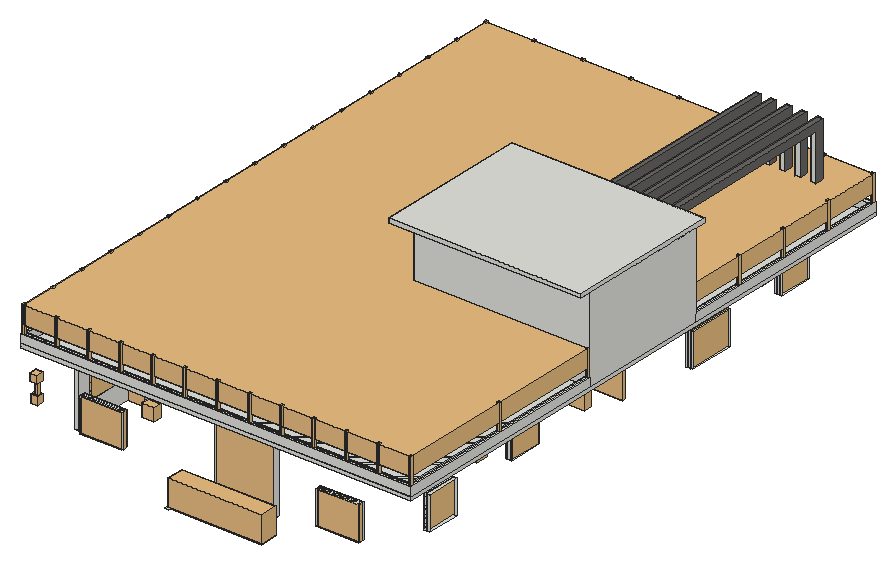
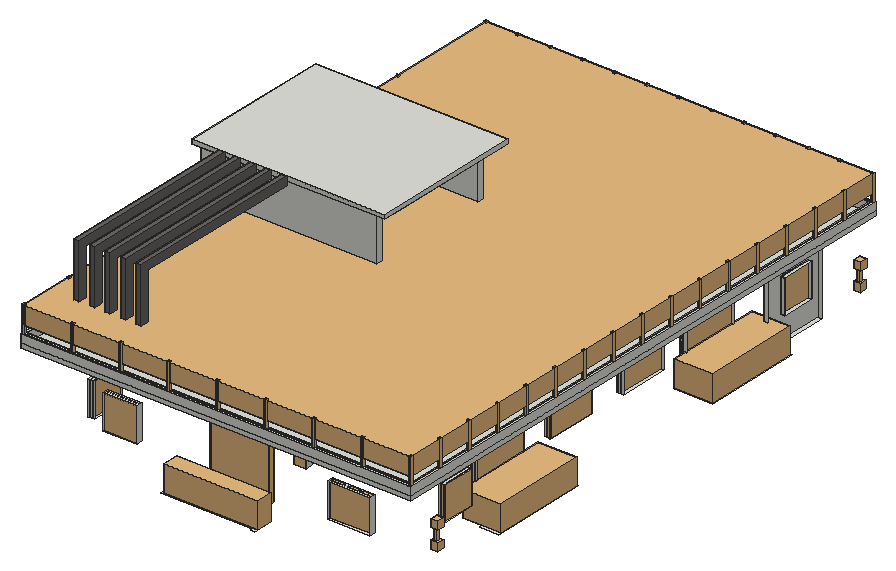
# SketchUp Ruby script. Lengths in inches.
U = 1.inch
M = Sketchup.active_model
def pt(a) = Geom::Point3d.new(a.map { |v| v * U })
def face(e, loops, mat)
  f = e.add_face(loops[0].map { |a| pt(a) })
  loops[1..].each { |l| e.add_face(l.map { |a| pt(a) }).erase! }
  f.material = f.back_material = mat if mat
  f
end
# faces: each face lists its corners as indices into pts; further lists are holes
def faces(e, pts, list, mat = nil) = list.each { |f| face(e, (f[0].is_a?(Array) ? f : [f]).map { |l| l.map { |i| pts[i] } }, mat) }
# xy, xz, yz: faces in a plane at the given z, y or x. An outline is a flat list of corners, or four numbers for a rectangle; further outlines are holes
def ring(l) = l.size == 4 ? [[l[0], l[1]], [l[2], l[1]], [l[2], l[3]], [l[0], l[3]]] : l.each_slice(2).to_a
def flat(e, list, mat, &to3) = list.each { |f| face(e, (f[0].is_a?(Array) ? f : [f]).map { |l| ring(l).map { |u, v| to3.(u, v) } }, mat) }
def xy(e, z, list, mat = nil) = flat(e, list, mat) { |x, y| [x, y, z] }
def xz(e, y, list, mat = nil) = flat(e, list, mat) { |x, z| [x, y, z] }
def yz(e, x, list, mat = nil) = flat(e, list, mat) { |y, z| [x, y, z] }
def lines(e, pts, list) = list.each { |a, b| e.add_line(pt(pts[a]), pt(pts[b])) }
# prism: a flat outline (further loops are holes) pulled along v
def prism(e, loops, v, mat = nil)
  f = face(e, loops, mat); d = Geom::Vector3d.new(v.map { |x| x * U })
  f.pushpull(f.normal.samedirection?(d) ? d.length : -d.length)
end
def box(e, o, s, mat = nil) = prism(e, [[o, [o[0] + s[0], o[1], o[2]], [o[0] + s[0], o[1] + s[1], o[2]], [o[0], o[1] + s[1], o[2]]]], [0, 0, s[2]], mat)
def at(x, y, z, deg = 0) = Geom::Transformation.translation(pt([x, y, z])) * Geom::Transformation.rotation(ORIGIN, Z_AXIS, deg.degrees)
def axes(o, x, y, z) = Geom::Transformation.new([*x, 0, *y, 0, *z, 0, *pt(o).to_a, 1])
def part(name) = M.definitions.add(name)
# library, detail: a bought-in or finely detailed component or shape, given as its bounding box
def library(name, o, s) = part(name).tap { |d| box(d.entities, o, s) }
def detail(e, o, s) = box(e.add_group.entities, o, s)
def put(e, d, t, mat = nil) = e.add_instance(d, t).tap { |i| i.material = mat if mat }
def group(e, t, mat = nil) = e.add_group.tap { |g| g.transformation = t; g.material = mat if mat }.entities
root = M.entities
M.materials.add("Stone C 250cm").color = [107, 104, 102]
c1 = library("Group\#21",[0,0,0],[134.45,23.44,36.98])
c2 = library("Window Crafter Sliding",[0,-0.55,0],[84,4.49,96])
c3 = library("Group\#18",[0,0,0],[54.77,134.11,36.98])
c4 = library("Group\#23",[0,0,0],[133.24,24.34,36.98])
c5 = library("Group\#17",[0,0,0],[54.54,138.15,36.98])
c6 = library("Group\#6",[0,0,0],[112.45,3.15,94.27])
c7 = library("Group\#11",[0,0,0],[103.79,11.15,157.27])
c8 = library("Window Crafter Sliding 6",[0,-0.55,0],[72,4.49,48])
c9 = library("Window Crafter Sliding 2",[0,-0.55,0],[48,4.49,48])
c10 = library("Window Crafter Sliding 5",[0,-0.55,0],[66,4.49,48])
c11 = library("Window Crafter Sliding 3",[0,-0.55,0],[60,4.49,48])
c12 = library("Spot Light\#1",[-5.1,-5.1,-11.05],[10.2,10.2,11.05])
c13 = library("Lamp Wall Outdoor 94-02",[-1.89,-4.65,-3.17],[3.78,4.65,6.35])
c14 = library("Group\#12",[0,0,0],[113.66,3.15,100.57])
c15 = library("Window Crafter Awning 2",[0,-9.5,0],[17.5,11.27,18])
c16 = library("Tlon Light 650 Ceiling 152 007",[-12.8,-12.8,-3.78],[25.6,25.6,3.58])
c17 = part("Square rail bar")
box(c17.entities,[0,0,-1],[51.7,1,1])
c18 = part("Group\#20")
xy(c18.entities,0,[[0,0,51.7,106.6]])
xy(c18.entities,1,[[0,0,51.7,107.6]])
xz(c18.entities,0,[[0,0,51.7,1]])
xz(c18.entities,107.6,[[0,0,51.7,1]])
yz(c18.entities,0,[[0,0,107.6,1]])
yz(c18.entities,51.7,[[0,0,107.6,1]])
put(c18.entities,c17,at(0,106.6,0))
put(c18.entities,c17,at(0,0,0))
put(c18.entities,c17,at(0,103.05,0))
put(c18.entities,c17,at(0,99.49,0))
put(c18.entities,c17,at(0,95.94,0))
put(c18.entities,c17,at(0,92.39,0))
put(c18.entities,c17,at(0,88.83,0))
put(c18.entities,c17,at(0,85.28,0))
put(c18.entities,c17,at(0,81.73,0))
put(c18.entities,c17,at(0,78.17,0))
put(c18.entities,c17,at(0,74.62,0))
put(c18.entities,c17,at(0,71.07,0))
put(c18.entities,c17,at(0,67.51,0))
put(c18.entities,c17,at(0,63.96,0))
put(c18.entities,c17,at(0,60.41,0))
put(c18.entities,c17,at(0,56.85,0))
put(c18.entities,c17,at(0,53.3,0))
put(c18.entities,c17,at(0,49.75,0))
put(c18.entities,c17,at(0,46.19,0))
put(c18.entities,c17,at(0,42.64,0))
put(c18.entities,c17,at(0,39.09,0))
put(c18.entities,c17,at(0,35.53,0))
put(c18.entities,c17,at(0,31.98,0))
put(c18.entities,c17,at(0,28.43,0))
put(c18.entities,c17,at(0,24.875,0))
put(c18.entities,c17,at(0,21.32,0))
put(c18.entities,c17,at(0,17.77,0))
put(c18.entities,c17,at(0,14.21,0))
put(c18.entities,c17,at(0,10.66,0))
put(c18.entities,c17,at(0,7.11,0))
put(c18.entities,c17,at(0,3.55,0))
put(c18.entities,c17,at(0,0,0))
c19 = part("Opening frame")
xy(c19.entities,0,[[0,0,7.4375,12]])
xy(c19.entities,114,[[0,-246.7,7.4375,0]])
xy(c19.entities,126,[[0,-246.7,7.4375,12]],"Stone C 250cm")
xz(c19.entities,-246.7,[[0,114,7.4375,126]])
xz(c19.entities,0,[[0,0,7.4375,114]])
xz(c19.entities,12,[[0,0,7.4375,126]],"Stone C 250cm")
yz(c19.entities,0,[[0,0,0,114,-246.7,114,-246.7,126,12,126,12,0]],"Stone C 250cm")
yz(c19.entities,7.4375,[[0,0,12,0,12,126,-246.7,126,-246.7,114,0,114]],"Stone C 250cm")
c20 = library("Ploe\#3",[2336.18,686.95,516],[3.15,3.15,37.57])
c21 = part("Group1621\#2")
put(c21.entities,c20,at(0,0,0))
put(c21.entities,c20,at(0,79.49,0))
put(c21.entities,c20,at(0,158.98,0))
put(c21.entities,c20,at(0,238.46,0))
put(c21.entities,c20,at(0,317.95,0))
put(c21.entities,c20,at(-68.83,317.95,0))
put(c21.entities,c20,at(-137.65,317.95,0))
put(c21.entities,c20,at(-206.47,317.95,0))
put(c21.entities,c20,at(-275.3,317.95,0))
put(c21.entities,c20,at(-344.125,317.95,0))
put(c21.entities,c20,at(-412.95,317.95,0))
put(c21.entities,c20,at(-481.77,317.95,0))
put(c21.entities,c20,at(-550.6,317.95,0))
put(c21.entities,c20,at(-550.6,266.57,0))
put(c21.entities,c20,at(-550.6,215.2,0))
put(c21.entities,c20,at(-550.6,163.83,0))
put(c21.entities,c20,at(-550.6,112.45,0))
put(c21.entities,c20,at(-550.6,61.08,0))
put(c21.entities,c20,at(-550.6,9.7,0))
put(c21.entities,c20,at(-550.6,-41.67,0))
put(c21.entities,c20,at(-550.6,-93.05,0))
put(c21.entities,c20,at(-550.6,-144.42,0))
put(c21.entities,c20,at(-550.6,-195.8,0))
put(c21.entities,c20,at(-550.6,-247.17,0))
put(c21.entities,c20,at(-550.6,-298.55,0))
put(c21.entities,c20,at(-550.6,-349.92,0))
put(c21.entities,c20,at(-550.6,-401.3,0))
put(c21.entities,c20,at(-550.6,-452.67,0))
put(c21.entities,c20,at(-550.6,-504.05,0))
put(c21.entities,c20,at(-504.72,-504.05,0))
put(c21.entities,c20,at(-458.83,-504.05,0))
put(c21.entities,c20,at(-412.95,-504.05,0))
put(c21.entities,c20,at(-367.07,-504.05,0))
put(c21.entities,c20,at(-321.18,-504.05,0))
put(c21.entities,c20,at(-275.3,-504.05,0))
put(c21.entities,c20,at(-229.42,-504.05,0))
put(c21.entities,c20,at(-183.53,-504.05,0))
put(c21.entities,c20,at(-137.65,-504.05,0))
put(c21.entities,c20,at(-91.77,-504.05,0))
put(c21.entities,c20,at(-45.88,-504.05,0))
put(c21.entities,c20,at(0,-504.05,0))
put(c21.entities,c20,at(0,-346.67,0))
put(c21.entities,c20,at(0,-189.3,0))
c22 = library("Group1622\#2",[1786.37,183.69,527.61],[552.17,823.58,25.18])
xy(root,381,[[2005.02,473.67,2011.02,473.67,2011.02,476.67,2141.52,476.67,2141.52,500.67,2138.32,500.67,2138.32,479.88,2008.23,479.88,2008.23,500.67,2005.02,500.67],[2008.23,479.88,2138.32,479.88,2138.32,500.67,2135.52,500.67,2135.52,482.67,2011.02,482.67,2011.02,500.67,2008.23,500.67],[2031.27,530.62,2115.27,539.67],[1789.02,637.17,1816.02,637.17,1816.02,640.17,1792.02,640.17,1792.02,775.17,1843.02,775.17,1843.02,778.17,1789.02,778.17],[1792.02,640.17,1816.02,640.17,1816.02,643.17,1795.02,643.17,1795.02,772.17,1843.02,772.17,1843.02,775.17,1792.02,775.17],
  [1843.02,673.67,1852.02,757.67],[1789.02,1018.17,1843.02,1018.17,1843.02,1020.95,1791.8,1020.95,1791.8,1151.9,1816.02,1151.9,1816.02,1159.17,1789.02,1159.17],[1791.8,1020.95,1843.02,1020.95,1843.02,1024.17,1795.02,1024.17,1795.02,1148.67,1816.02,1148.67,1816.02,1151.9,1791.8,1151.9],[1843.02,1046.67,1852.02,1130.67],[2031.27,1256.67,2115.27,1265.67],
  [2005.02,1295.67,2011.02,1295.67,2011.02,1313.67,2135.52,1313.67,2135.52,1295.67,2141.52,1295.67,2141.52,1319.67,2011.02,1319.67,2011.02,1322.67,2005.02,1322.67],[2007.35,1298.57,2007.22,1298.59,2007.1,1298.64,2007,1298.72,2006.92,1298.82,2006.87,1298.94,2006.85,1299.07,2006.87,1299.2,2006.92,1299.32,2007,1299.42,2007.1,1299.5,2007.22,1299.55,2007.35,1299.57,2007.48,1299.55,2007.6,1299.5,2007.7,1299.42,2007.78,1299.32,2007.83,1299.2,2007.85,1299.07,2007.83,1298.94,2007.78,1298.82,2007.7,1298.72,2007.6,1298.64,2007.48,1298.59],[2007.35,1315.07,2007.22,1315.09,2007.1,1315.14,2007,1315.22,2006.92,1315.32,2006.87,1315.44,2006.85,1315.57,2006.87,1315.7,2006.92,1315.82,2007,1315.92,2007.1,1316,2007.22,1316.05,2007.35,1316.07,2007.48,1316.05,2007.6,1316,2007.7,1315.92,2007.78,1315.82,2007.83,1315.7,2007.85,1315.57,2007.83,1315.44,2007.78,1315.32,2007.7,1315.22,2007.6,1315.14,2007.48,1315.09],[2051.11,1315.07,2050.98,1315.09,2050.86,1315.14,2050.76,1315.22,2050.68,1315.32,2050.63,1315.44,2050.61,1315.57,2050.63,1315.7,2050.68,1315.82,2050.76,1315.92,2050.86,1316,2050.98,1316.05,2051.11,1316.07,2051.24,1316.05,2051.36,1316,2051.47,1315.92,2051.55,1315.82,2051.6,1315.7,2051.61,1315.57,2051.6,1315.44,2051.55,1315.32,2051.47,1315.22,2051.36,1315.14,2051.24,1315.09],[2138.64,1315.07,2138.52,1315.09,2138.39,1315.14,2138.29,1315.22,2138.21,1315.32,2138.16,1315.44,2138.14,1315.57,2138.16,1315.7,2138.21,1315.82,2138.29,1315.92,2138.39,1316,2138.52,1316.05,2138.64,1316.07,2138.77,1316.05,2138.89,1316,2139,1315.92,2139.08,1315.82,2139.13,1315.7,2139.14,1315.57,2139.13,1315.44,2139.08,1315.32,2139,1315.22,2138.89,1315.14,2138.77,1315.09]])
xy(root,381.02,[[1815.02,551.67,1820.92,647.67]])
xy(root,414,[[1863.02,500.67,1923.02,509.67],[2199.52,500.67,2259.52,509.67],[1815.02,569.57,1820.92,617.57],[1816.02,569.57,1825.02,617.57],[2297.52,569.57,2306.52,617.57],
  [2267.52,752.67,2276.52,800.67],[1843.02,797.67,1852.02,869.67],[1843.02,926.67,1852.02,998.67],[2294.52,1040.67,2303.52,1106.67],[1816.02,1172.67,1825.02,1220.67],
  [2267.52,1232.67,2276.52,1280.67],[1863.02,1286.67,1923.02,1295.67],[2195.52,1286.67,2243.52,1295.67]])
xy(root,462,[[1863.02,500.67,1923.02,509.67],[2199.52,500.67,2259.52,509.67],[1815.02,569.57,1820.92,617.57],[1816.02,569.57,1825.02,617.57],[2297.52,569.57,2306.52,617.57],
  [1954.02,596.67,1978.02,602.67],[2005.02,605.67,2011.02,635.67],[2152.02,641.67,2184.02,647.67],[2198.52,641.67,2228.52,647.67],[2267.52,710.67,2276.52,740.67],
  [2267.52,752.67,2276.52,800.67],[1966.02,767.67,2002.02,773.67],[1843.02,797.67,1852.02,869.67],[2078.52,806.67,2117.52,815.67],[2008.02,809.67,2014.02,833.67],
  [1843.02,926.67,1852.02,998.67],[2008.02,962.67,2014.02,986.67],[2078.52,980.67,2117.52,989.67],[1966.02,1022.67,2002.02,1028.67],[2294.52,1040.67,2303.52,1106.67],
  [2149.02,1121.67,2181.02,1127.67],[2195.52,1121.67,2225.52,1127.67],[2005.02,1160.17,2011.02,1190.17],[1816.02,1172.67,1825.02,1220.67],[2267.52,1190.67,2276.52,1220.67],
  [1954.02,1193.67,1978.02,1199.67],[2267.52,1232.67,2276.52,1280.67],[1863.02,1286.67,1923.02,1295.67],[2195.52,1286.67,2243.52,1295.67]])
xy(root,468,[[1953.02,500.67,1970.52,509.67],[2297.52,649.73,2306.52,667.23],[2029.77,869.67,2047.27,878.67],[2029.77,917.67,2047.27,926.67],[2294.52,1162.17,2303.52,1179.67],
  [1953.02,1286.67,1970.52,1295.67]])
xy(root,477,[[2031.27,530.62,2115.27,539.67],[1843.02,673.67,1852.02,757.67],[1843.02,1046.67,1852.02,1130.67],[2031.27,1256.67,2115.27,1265.67]])
xy(root,486,[[1953.02,500.67,1970.52,509.67],[2297.52,649.73,2306.52,667.23],[2029.77,869.67,2047.27,878.67],[2029.77,917.67,2047.27,926.67],[2294.52,1162.17,2303.52,1179.67],
  [1953.02,1286.67,1970.52,1295.67]])
xy(root,498,[[[1789.02,500.67,2011.02,500.67,2011.02,647.67,1852.02,647.67,1852.02,767.67,2072.52,767.67,2072.52,806.67,2132.52,806.67,2132.52,715.17,2066.52,715.17,2066.52,686.67,2072.52,686.67,2072.52,709.17,2132.52,709.17,2132.52,686.67,2138.52,686.67,2138.52,743.67,2158.52,743.67,2158.52,749.67,2138.52,749.67,2138.52,806.67,2324.52,806.67,2324.52,815.67,2276.52,815.67,2276.52,980.67,2330.52,980.67,2330.52,1031.67,2303.52,1031.67,2303.52,1151.7,2324.52,1151.7,2324.52,1157.7,2303.52,1157.7,2303.52,1181.67,2330.52,1181.67,2330.52,1295.67,2132.52,1295.67,2132.52,1223.67,2138.52,1223.67,2138.52,1286.67,2324.52,1286.67,2324.52,1187.67,2132.52,1187.67,2132.52,1181.67,2183.52,1181.67,2183.52,1127.67,2132.52,1127.67,2132.52,989.67,2072.52,989.67,2072.52,1028.67,1852.02,1028.67,1852.02,1148.67,2011.02,1148.67,2011.02,1256.67,2132.52,1256.67,2132.52,1265.67,2011.02,1265.67,2011.02,1295.67,1798.02,1295.67,1798.02,1286.67,1945.02,1286.67,1945.02,1193.67,2005.02,1193.67,2005.02,1157.67,1997.02,1157.67,1997.02,1154.67,1825.02,1154.67,1825.02,1253.67,1816.02,1253.67,1816.02,1148.67,1843.02,1148.67,1843.02,647.67,1816.02,647.67,1816.02,551.67,1789.02,551.67],[1852.02,773.67,1852.02,893.67,2014.02,893.67,2014.02,891.17,2017.02,891.17,2017.02,905.17,2014.02,905.17,2014.02,902.67,1852.02,902.67,1852.02,1022.67,2008.02,1022.67,2008.02,902.67,2014.02,902.67,2014.02,1022.67,2066.52,1022.67,2066.52,773.67,2014.02,773.67,2014.02,893.67,2008.02,893.67,2008.02,773.67],[2075.52,815.67,2267.52,980.67],[1798.02,509.67,1798.02,542.67,1825.02,542.67,1825.02,641.67,1997.02,641.67,1997.02,638.67,2005.02,638.67,2005.02,509.67],[2138.52,989.67,2138.52,1118.67,2146.52,1118.67,2146.52,1121.67,2294.52,1121.67,2294.52,1022.67,2321.52,1022.67,2321.52,989.67],[2189.52,1127.67,2294.52,1181.67],[1951.02,1199.67,2005.02,1286.67]],[[2135.52,500.67,2333.52,500.67,2333.52,551.67,2306.52,551.67,2306.52,701.67,2333.52,701.67,2333.52,806.67,2327.52,806.67,2327.52,707.67,2186.52,707.67,2186.52,647.67,2135.52,647.67,2135.52,539.67,2011.02,539.67,2011.02,530.62,2135.52,530.62],[2141.52,509.67,2141.52,641.67,2297.52,641.67,2297.52,542.67,2324.52,542.67,2324.52,509.67],[2192.52,647.67,2297.52,701.67]],[1945.02,509.67,1951.02,509.67,1951.02,596.67,2005.02,596.67,2005.02,602.67,1945.02,602.67],[1815.02,551.67,1820.92,647.67],[2267.52,707.67,2276.52,806.67],
  [2324.52,806.67,2333.52,815.67],[2014.02,869.67,2066.52,878.67],[2014.02,917.67,2066.52,926.67],[2066.52,1081.17,2132.52,1081.17,2132.52,1087.17,2072.52,1087.17,2072.52,1109.67,2066.52,1109.67],[2132.52,1157.67,2138.52,1181.67],
  [2267.52,1187.67,2276.52,1286.67],[1789.02,1244.67,1816.02,1244.67,1816.02,1253.67,1798.02,1253.67,1798.02,1295.67,1789.02,1295.67]])
xy(root,504,[[1782.92,494.57,1782.92,1322.67,2339.625,1322.67,2339.625,1001.67,2333.52,1001.67,2333.52,1316.67,1788.92,1316.67,1788.92,500.57,2333.52,500.57,2333.52,812.375,2339.625,812.375,2339.625,494.57],[[1788.92,500.57,2333.52,500.57,2333.52,812.375,2088.94,812.375,2088.94,821.375,2324.52,821.375,2324.52,992.67,2088.94,992.67,2088.94,1001.67,2333.52,1001.67,2333.52,1316.67,1788.92,1316.67],[2128.52,887.07,2267.52,980.67]],[2088.94,812.375,2088.94,821.375,2324.52,821.375,2324.52,992.67,2088.94,992.67,2088.94,1001.67,2339.625,1001.67,2339.625,812.375]])
xy(root,516,[[1782.92,494.57,2339.625,494.57,2339.625,812.375,2336.57,812.375,2336.57,497.625,1785.97,497.625,1785.97,1319.625,2336.57,1319.625,2336.57,1001.67,2339.625,1001.67,2339.625,1322.67,1782.92,1322.67],[1785.97,497.625,2336.57,497.625,2336.57,812.375,2333.52,812.375,2333.52,500.57,1788.92,500.57,1788.92,1316.67,2333.52,1316.67,2333.52,1001.67,2336.57,1001.67,2336.57,1319.625,1785.97,1319.625]])
xy(root,624,[[2064.94,797.375,2339.625,812.375],[2064.94,812.375,2088.94,821.375],[2088.94,812.375,2339.625,821.375],[2064.94,821.375,2324.52,992.67],[2324.52,821.375,2339.625,992.67],
  [2064.94,992.67,2088.94,1001.67],[2088.94,992.67,2339.625,1001.67],[2064.94,1001.67,2339.625,1016.67]])
xy(root,630,[[2064.94,797.375,2339.625,1016.67]])
xz(root,494.57,[[1782.92,504,2339.625,516]])
xz(root,500.57,[[1788.92,504,2333.52,516]])
xz(root,551.67,[[1815.02,381.02,1820.92,498]])
xz(root,569.57,[[1815.02,414,1820.92,462],[1816.02,414,1825.02,462],[2297.52,414,2306.52,462]])
xz(root,617.57,[[1815.02,414,1820.92,462],[1816.02,414,1825.02,462],[2297.52,414,2306.52,462]])
xz(root,647.67,[[1815.02,381.02,1820.92,498]])
xz(root,649.73,[[2297.52,468,2306.52,486]])
xz(root,667.23,[[2297.52,468,2306.52,486]])
xz(root,673.67,[[1843.02,381,1852.02,477]])
xz(root,752.67,[[2267.52,414,2276.52,462]])
xz(root,757.67,[[1843.02,381,1852.02,477]])
xz(root,797.375,[[2064.94,624,2339.625,630]])
xz(root,797.67,[[1843.02,414,1852.02,462]])
xz(root,800.67,[[2267.52,414,2276.52,462]])
xz(root,812.375,[[2088.94,504,2333.52,504,2333.52,516,2339.625,516,2339.625,624,2088.94,624],[2333.52,504,2339.625,516]])
xz(root,821.375,[[2088.94,504,2324.52,624]])
xz(root,869.67,[[1843.02,414,1852.02,462]])
xz(root,926.67,[[1843.02,414,1852.02,462]])
xz(root,992.67,[[2088.94,504,2324.52,624]])
xz(root,998.67,[[1843.02,414,1852.02,462]])
xz(root,1001.67,[[2088.94,504,2088.94,624,2339.625,624,2339.625,516,2333.52,516,2333.52,504],[2333.52,504,2339.625,516]])
xz(root,1016.67,[[2064.94,624,2205.125,630],[2205.125,624,2301.125,630],[2301.125,624,2339.625,630]])
xz(root,1040.67,[[2294.52,414,2303.52,462]])
xz(root,1046.67,[[1843.02,381,1852.02,477]])
xz(root,1106.67,[[2294.52,414,2303.52,462]])
xz(root,1130.67,[[1843.02,381,1852.02,477]])
xz(root,1162.17,[[2294.52,468,2303.52,486]])
xz(root,1172.67,[[1816.02,414,1825.02,462]])
xz(root,1179.67,[[2294.52,468,2303.52,486]])
xz(root,1220.67,[[1816.02,414,1825.02,462]])
xz(root,1232.67,[[2267.52,414,2276.52,462]])
xz(root,1280.67,[[2267.52,414,2276.52,462]])
xz(root,1316.67,[[1788.92,504,2333.52,516]])
xz(root,1322.67,[[1782.92,504,2339.625,516]])
yz(root,1782.92,[[494.57,504,1322.67,516]])
yz(root,1788.92,[[500.57,504,1316.67,516]])
yz(root,1820.92,[[551.67,381.02,647.67,498],[569.57,414,617.57,462]])
yz(root,1863.02,[[500.67,414,509.67,462],[1286.67,414,1295.67,462]])
yz(root,1923.02,[[500.67,414,509.67,462],[1286.67,414,1295.67,462]])
yz(root,1953.02,[[500.67,468,509.67,486],[1286.67,468,1295.67,486]])
yz(root,1970.52,[[500.67,468,509.67,486],[1286.67,468,1295.67,486]])
yz(root,2029.77,[[869.67,468,878.67,486],[917.67,468,926.67,486]])
yz(root,2031.27,[[530.62,381,539.67,477],[1256.67,381,1265.67,477]])
yz(root,2047.27,[[869.67,468,878.67,486],[917.67,468,926.67,486]])
yz(root,2064.94,[[797.375,624,1016.67,630]])
yz(root,2088.94,[[812.375,504,821.375,624],[992.67,504,1001.67,624]])
yz(root,2115.27,[[530.62,381,539.67,477],[1256.67,381,1265.67,477]])
yz(root,2195.52,[[1286.67,414,1295.67,462]])
yz(root,2199.52,[[500.67,414,509.67,462]])
yz(root,2243.52,[[1286.67,414,1295.67,462]])
yz(root,2259.52,[[500.67,414,509.67,462]])
yz(root,2324.52,[[821.375,504,992.67,624]])
yz(root,2333.52,[[500.57,504,812.375,516],[1001.67,504,1316.67,516]])
yz(root,2339.625,[[494.57,504,812.375,516],[812.375,504,1001.67,624],[1001.67,504,1322.67,516],[797.375,624,1016.67,630]])
p = [[1794.67,506.67,503.75],[1794.67,506.67,504],[2100.0625,1316,381],[2100.17,1315.92,381],[2099.33,1315.44,381],[2099.3125,1315.57,381],
  [2099.33,1315.7,381],[2099.38,1315.82,381],[2099.46,1315.92,381],[2099.5625,1316,381],[2099.68,1316.05,381],[2099.8125,1316.07,381],
  [2099.94,1316.05,381],[2100.25,1315.82,381],[2100.3,1315.7,381],[2100.3125,1315.57,381],[2100.3,1315.44,381],[2100.25,1315.32,381],
  [2100.17,1315.22,381],[2100.0625,1315.14,381],[2099.94,1315.09,381],[2099.8125,1315.07,381],[2099.68,1315.09,381],[2099.5625,1315.14,381],
  [2099.46,1315.22,381],[2099.38,1315.32,381],[1816.02,1148.61,381],[1795.09,1148.61,381],[1795.09,1024.24,381],[1843.02,1024.24,381],
  [1816.02,1148.51,381],[1795.1875,1148.51,381],[1795.1875,1024.34,381],[1843.02,1024.34,381]]
lines(root,p,[[0,1],[2,3],[4,5],[5,6],[6,7],[7,8],[8,9],[9,10],[10,11],[11,12],[12,2],[3,13],
  [13,14],[14,15],[15,16],[16,17],[17,18],[18,19],[19,20],[20,21],[21,22],[22,23],[23,24],[24,25],
  [25,4],[26,27],[27,28],[28,29],[30,31],[31,32],[32,33]])
put(root,c1,at(2005.77,1293.7,381))
put(root,c2,at(2031.27,533.26,381))
put(root,c2,at(1849.22,1046.67,381,90))
put(root,c2,at(2031.27,1259.48,381))
put(root,c2,at(1851.46,673.67,381,90))
put(root,c3,at(1790.22,1019.37,381))
put(root,c4,at(2006.65,478.3,381))
put(root,c5,at(1790.45,638.6,381))
put(root,c6,at(2142.15,978.1,384.3))
put(root,c7,at(2131.95,933.1,384.3))
put(root,c8,at(1844.98,998.67,414,-90))
put(root,c9,at(2270.52,1280.67,414,-90))
put(root,c9,at(1818.83,1220.67,414,-90))
put(root,c8,at(1847.52,869.67,414,-90))
put(root,c10,at(2300.72,1040.67,414,90))
put(root,c11,at(2199.52,503.48,414))
put(root,c9,at(1820.52,617.57,414,-90))
put(root,c11,at(1863.02,503.48,414))
put(root,c9,at(2270.52,800.67,414,-90))
put(root,c11,at(1863.02,1287.79,414))
put(root,c9,at(2297.52,617.57,414,-90))
put(root,c9,at(2243.52,1293.71,414,180))
put(root,c12,at(1784.03,1275.46,427.42))
put(root,c12,at(1784.03,522.625,427.42))
put(root,c13,axes([1787.14,1275.32,435.66],[0,-1,0],[1,0,0],[0,0,2.6448]))
put(root,c13,axes([1787.14,522.48,435.66],[0,-1,0],[1,0,0],[0,0,2.6448]))
put(root,c14,at(2131.95,896.1,441))
put(root,c12,axes([1783.68,1275.18,443.94],[1,0,0],[0,1,0],[0,0,-1]))
put(root,c12,axes([1783.68,522.34,443.94],[1,0,0],[0,1,0],[0,0,-1]))
put(root,c15,at(2029.77,924.9,468))
put(root,c15,at(2047.27,869.67,468,180))
put(root,c15,at(2296.3,1162.17,468,90))
put(root,c15,at(1970.52,1288.45,468,180))
put(root,c15,at(2299.3,649.73,468,90))
put(root,c15,at(1953.02,507.9,468))
put(root,c16,axes([1817.33,679.8,496.04],[0.44,0,0],[0,0.44,0],[0,0,0.44]))
put(root,c16,axes([1817.33,726,496.04],[0.44,0,0],[0,0.44,0],[0,0,0.44]))
put(root,c16,axes([2034,1282.86,496.21],[0.44,0,0],[0,0.44,0],[0,0,0.44]))
put(root,c16,axes([2077.86,1282.86,496.21],[0.44,0,0],[0,0.44,0],[0,0,0.44]))
put(root,c16,axes([1817.33,1048.52,496.24],[0.44,0,0],[0,0.44,0],[0,0,0.44]))
put(root,c16,axes([1817.33,1094.72,496.24],[0.44,0,0],[0,0.44,0],[0,0,0.44]))
put(root,c18,axes([1791.32,664.67,496.8],[1,0,0],[0,0.72,0],[0,0,1]))
put(root,c18,at(1791.32,1022.61,497))
put(root,c18,axes([2011.02,1301.77,497],[0,-0.69826,0],[0.97119,0,0],[0,0,1]))
g1 = group(root,at(1789.02,500.67,498))
prism(g1,[[[550.6,822,0],[550.6,-6.1,0],[-6.1,-6.1,0],[-6.1,822,0]],[[339.5,386.4,0],[478.5,386.4,0],[478.5,480,0],[339.5,480,0]]],[0,0,6])
put(root,c19,at(2293.6875,1263.375,504))
put(root,c19,at(2271.55,1263.375,504))
put(root,c19,at(2249.4,1263.375,504))
put(root,c19,at(2227.26,1263.375,504))
put(root,c19,at(2205.125,1263.375,504))
g2 = group(root,at(1784.4,496.05,516))
put(g2,c21,at(-1785.58,-182.9,-516))
put(g2,c22,at(-1785.58,-182.9,-516))
